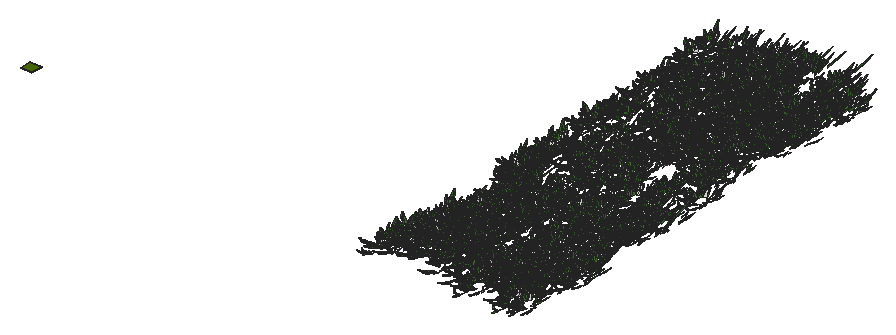
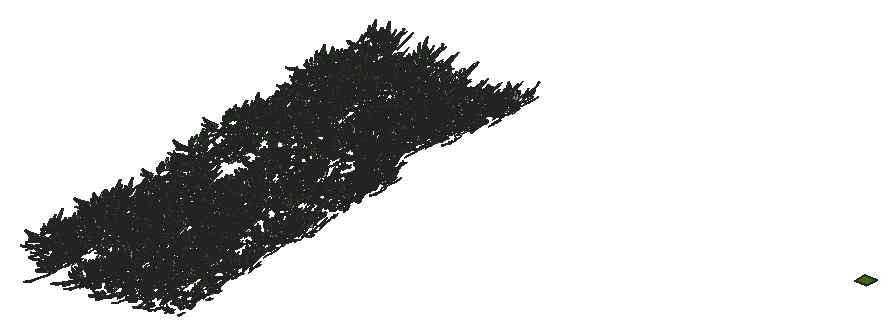
# SketchUp Ruby script. Lengths in inches.
U = 1.inch
M = Sketchup.active_model
def pt(a) = Geom::Point3d.new(a.map { |v| v * U })
def face(e, loops, mat)
  f = e.add_face(loops[0].map { |a| pt(a) })
  loops[1..].each { |l| e.add_face(l.map { |a| pt(a) }).erase! }
  f.material = f.back_material = mat if mat
  f
end
# faces: each face lists its corners as indices into pts; further lists are holes
def faces(e, pts, list, mat = nil) = list.each { |f| face(e, (f[0].is_a?(Array) ? f : [f]).map { |l| l.map { |i| pts[i] } }, mat) }
# xy, xz, yz: faces in a plane at the given z, y or x. An outline is a flat list of corners, or four numbers for a rectangle; further outlines are holes
def ring(l) = l.size == 4 ? [[l[0], l[1]], [l[2], l[1]], [l[2], l[3]], [l[0], l[3]]] : l.each_slice(2).to_a
def flat(e, list, mat, &to3) = list.each { |f| face(e, (f[0].is_a?(Array) ? f : [f]).map { |l| ring(l).map { |u, v| to3.(u, v) } }, mat) }
def xy(e, z, list, mat = nil) = flat(e, list, mat) { |x, y| [x, y, z] }
def xz(e, y, list, mat = nil) = flat(e, list, mat) { |x, z| [x, y, z] }
def yz(e, x, list, mat = nil) = flat(e, list, mat) { |y, z| [x, y, z] }
def lines(e, pts, list) = list.each { |a, b| e.add_line(pt(pts[a]), pt(pts[b])) }
# prism: a flat outline (further loops are holes) pulled along v
def prism(e, loops, v, mat = nil)
  f = face(e, loops, mat); d = Geom::Vector3d.new(v.map { |x| x * U })
  f.pushpull(f.normal.samedirection?(d) ? d.length : -d.length)
end
def box(e, o, s, mat = nil) = prism(e, [[o, [o[0] + s[0], o[1], o[2]], [o[0] + s[0], o[1] + s[1], o[2]], [o[0], o[1] + s[1], o[2]]]], [0, 0, s[2]], mat)
def at(x, y, z, deg = 0) = Geom::Transformation.translation(pt([x, y, z])) * Geom::Transformation.rotation(ORIGIN, Z_AXIS, deg.degrees)
def axes(o, x, y, z) = Geom::Transformation.new([*x, 0, *y, 0, *z, 0, *pt(o).to_a, 1])
def part(name) = M.definitions.add(name)
# library, detail: a bought-in or finely detailed component or shape, given as its bounding box
def library(name, o, s) = part(name).tap { |d| box(d.entities, o, s) }
def detail(e, o, s) = box(e.add_group.entities, o, s)
def put(e, d, t, mat = nil) = e.add_instance(d, t).tap { |i| i.material = mat if mat }
def group(e, t, mat = nil) = e.add_group.tap { |g| g.transformation = t; g.material = mat if mat }.entities
root = M.entities
M.materials.add("Material10").color = [48, 90, 38]
M.materials.add("Material11").color = [68, 110, 48]
M.materials.add("Material12").color = [48, 90, 48]
M.materials.add("Material13").color = [58, 110, 58]
M.materials.add("Material14").color = [58, 90, 38]
M.materials.add("Material15").color = [68, 100, 58]
M.materials.add("Material16").color = [48, 100, 38]
M.materials.add("Material9").color = [68, 110, 58]
M.materials.add("[Groundcover_BarkChips]").color = [80, 57, 35]
M.materials.add("[Groundcover_RiverRock_4inch]").color = [80, 57, 35]
M.materials.add("[Groundcover_Rock_Crushed_2inch]").color = [74, 111, 8]
c1 = part("Untitled")
xy(c1.entities,0.3125,[[-290.45,43.1875,-283.67,49.67]],"[Groundcover_RiverRock_4inch]")
xy(c1.entities,0.6875,[[-290.45,43.1875,-283.67,49.67]],"[Groundcover_Rock_Crushed_2inch]")
xz(c1.entities,43.1875,[[-290.45,0.3125,-283.67,0.6875]],"[Groundcover_BarkChips]")
xz(c1.entities,49.67,[[-290.45,0.3125,-283.67,0.6875]],"[Groundcover_BarkChips]")
yz(c1.entities,-290.45,[[43.1875,0.3125,49.67,0.6875]],"[Groundcover_BarkChips]")
yz(c1.entities,-283.67,[[43.1875,0.3125,49.67,0.6875]],"[Groundcover_BarkChips]")
c2 = part("grass00")
p = [[-0.6875,0.15,0],[-0.56,0.08,5.52],[-0.04,0.03,2.76],[0.48,-0.02,0],[0.35,-0.02,5.52],[-0.1,-0.14,5.52],
  [-0.12,0.65,8.37],[-0.42,0.65,8.37]]
faces(c2.entities,p,[[0,1,2,3],[3,2,4],[1,5,2],[5,4,2],[1,6,5],[4,5,6],[7,6,1]])
c3 = part("Group16\#1")
put(c3.entities,c2,axes([1.44,-0.61,-0.01],[0.05352,0.12609,0],[-0.10704,0.04543,0.07239],[0.06664,-0.02828,0.11628]),"Material12")
put(c3.entities,c2,axes([0.76,-0.15,-0.01],[0.04676,0.24062,0],[-0.23162,0.04501,0.06642],[0.0652,-0.01267,0.23595]),"Material9")
put(c3.entities,c2,axes([0.79,0.01,-0.01],[-0.00606,0.34651,0],[-0.34381,-0.00602,0.0432],[0.04319,0.00076,0.34386]))
put(c3.entities,c2,axes([1,0.23,-0.01],[-0.07192,0.31144,0],[-0.28722,-0.06632,0.1236],[0.12043,0.02781,0.29478]),"Material11")
put(c3.entities,c2,axes([1.66,0.77,-0.01],[-0.13828,0.29651,0],[-0.21551,-0.1005,0.22471],[0.20365,0.09498,0.23779]),"Material16")
put(c3.entities,c2,axes([0.6875,0.52,-0.01],[-0.18126,0.24051,0],[-0.22746,-0.17142,0.09788],[0.07817,0.05891,0.28481]),"Material11")
put(c3.entities,c2,axes([0.68,0.78,-0.01],[-0.215,0.18688,0],[-0.12385,-0.14248,0.21334],[0.13995,0.16101,0.18878]),"Material9")
put(c3.entities,c2,axes([0.56,1,-0.01],[-0.13756,0.07624,0],[-0.06159,-0.11112,0.0927],[0.04494,0.08108,0.12705]),"Material11")
put(c3.entities,c2,axes([0.2,0.64,-0.01],[-0.23729,0.07254,0],[-0.05711,-0.18681,0.153],[0.04473,0.14632,0.19535]),"Material16")
put(c3.entities,c2,axes([0.0625,0.72,-0.01],[-0.28874,0.02525,0],[-0.02179,-0.24916,0.14647],[0.01276,0.14591,0.25012]),"Material9")
put(c3.entities,c2,axes([-0.08,0.62,-0.01],[-0.34089,-0.04187,0],[0.03255,-0.26504,0.216],[-0.02633,0.21439,0.26703]),"Material16")
put(c3.entities,c2,axes([-0.34,0.98,-0.01],[-0.14314,-0.0493,0],[0.04397,-0.12769,0.06843],[-0.02228,0.0647,0.13505]),"Material16")
put(c3.entities,c2,axes([-0.87,1.45,-0.01],[-0.23488,-0.14114,0],[0.13761,-0.22901,0.06087],[-0.03135,0.05217,0.26717]))
put(c3.entities,c2,axes([-0.72,0.77,-0.01],[-0.14208,-0.13251,0],[0.07209,-0.0773,0.16301],[-0.11118,0.11922,0.1057]),"Material16")
put(c3.entities,c2,axes([-0.62,0.43,-0.01],[-0.14845,-0.21203,0],[0.18654,-0.13061,0.12304],[-0.10079,0.07057,0.22772]),"Material9")
put(c3.entities,c2,axes([-0.68,0.29,-0.01],[-0.13639,-0.32136,0],[0.31723,-0.13464,0.05579],[-0.05136,0.0218,0.34462]),"Material10")
put(c3.entities,c2,axes([-0.64,0.125,-0.01],[-0.0458,-0.23569,0],[0.22124,-0.043,0.08276],[-0.08124,0.01579,0.22538]),"Material13")
put(c3.entities,c2,axes([-1.6,-0.03,-0.01],[0.00576,-0.32897,0],[0.27526,0.00482,0.18018],[-0.18015,-0.00315,0.2753]),"Material11")
put(c3.entities,c2,axes([-1.36,-0.31,-0.01],[0.05718,-0.24765,0],[0.18172,0.04196,0.17267],[-0.16825,-0.03885,0.1865]),"Material16")
put(c3.entities,c2,axes([-1.54,-0.72,-0.01],[0.06537,-0.14017,0],[0.13555,0.06321,0.03939],[-0.0357,-0.01665,0.14956]))
put(c3.entities,c2,axes([-1.19,-0.9,-0.01],[0.09597,-0.12735,0],[0.11214,0.08451,0.07557],[-0.06035,-0.04548,0.14042]),"Material15")
put(c3.entities,c2,axes([-0.47,-0.54,-0.01],[0.11588,-0.10072,0],[0.0618,0.0711,0.12124],[-0.07953,-0.0915,0.0942]))
put(c3.entities,c2,axes([-0.47,-0.84,-0.01],[0.11927,-0.0661,0],[0.06603,0.11913,0.00646],[-0.00313,-0.00565,0.13621]),"Material11")
put(c3.entities,c2,axes([-0.38,-1.24,-0.01],[0.28037,-0.08571,0],[0.0618,0.20215,0.20315],[-0.05939,-0.19428,0.21139]),"Material15")
put(c3.entities,c2,axes([-0.06,-0.66,-0.01],[0.22719,-0.01987,0],[0.01247,0.14255,0.17758],[-0.01547,-0.17691,0.1431]),"Material14")
put(c3.entities,c2,axes([0.11,-0.89,-0.01],[0.14882,0.01828,0],[-0.01058,0.08611,0.12229],[0.01491,-0.12138,0.08676]),"Material12")
put(c3.entities,c2,axes([0.25,-0.72,-0.01],[0.20481,0.07053,0],[-0.06206,0.18022,0.10291],[0.03351,-0.0973,0.1906]),"Material12")
put(c3.entities,c2,axes([0.85,-1.42,-0.01],[0.16481,0.09904,0],[-0.09472,0.15762,0.05616],[0.02893,-0.04814,0.18389]),"Material11")
put(c3.entities,c2,axes([1.01,-1.09,-0.01],[0.21858,0.20385,0],[-0.17495,0.1876,0.15339],[0.10462,-0.11218,0.25652]),"Material16")
put(c3.entities,c2,axes([1.01,-0.71,-0.01],[0.08733,0.12473,0],[-0.06445,0.04512,0.13037],[0.1068,-0.07477,0.07867]),"Material12")
c4 = part("Group15\#1")
put(c4.entities,c3,at(0,0,0))
c5 = part("3darcstudiotree_grass00\#1")
put(c5.entities,c4,at(0,0,0))
put(root,c1,at(865.12,488.43,12.75))
put(root,c5,axes([800.23,508.89,12.99],[2.09672,-5.29532,0],[2.32944,4.81953,-0.01132],[0.03564,0.07375,1.83032]))
put(root,c5,axes([800.95,655.86,12.99],[0.31946,-6.70792,0],[3.10987,0.77388,-0.01362],[0.04886,0.01216,1.54899]))
put(root,c5,axes([801.36,701.5,12.99],[-1.12933,-6.15608,0],[2.41129,-2.31138,-0.00949],[0.03992,-0.03827,1.63563]))
put(root,c5,axes([800.76,739.52,12.99],[-1.09212,5.80129,0],[-2.59208,-2.54976,-0.01574],[-0.06215,-0.06113,1.66349]))
put(root,c5,axes([801.09,602.27,12.99],[2.14192,-4.884,0],[1.79828,4.12087,-0.0036],[0.0115,0.02635,1.5794]))
put(root,c5,axes([801.25,727.03,12.99],[-1.91744,4.33181,0],[-2.27081,-5.25216,-0.01852],[-0.0442,-0.10223,1.50457]))
put(root,c5,axes([801.03,526.67,12.99],[2.9199,-1.29353,0],[0.61218,7.22061,-0.01483],[0.00967,0.114,1.51152]))
put(root,c5,axes([802.77,513.77,12.99],[3.12278,0.02412,0],[-0.00853,5.77007,-0.00416],[-0.00005,0.03676,1.3392]))
put(root,c5,axes([804.21,703.32,12.99],[-0.82802,-6.3908,0],[2.45507,-1.66208,-0.01669],[0.08291,-0.05613,1.82011]))
put(root,c5,axes([804.46,691.14,12.99],[-2.76923,-1.21771,0],[0.5023,-5.96879,-0.01319],[0.01203,-0.14291,1.76124]))
put(root,c5,axes([804.6875,601.86,12.99],[1.26765,-5.25445,0],[2.71341,3.42052,-0.00061],[0.00243,0.00307,1.94394]))
put(root,c5,axes([804.25,627.625,12.99],[-1.44997,6.09404,0],[-2.85681,-3.55173,-0.01158],[-0.03373,-0.04193,1.47884]))
put(root,c5,axes([805.29,654.14,12.99],[-0.35039,-7.84154,0],[2.81713,-0.65775,-0.01024],[0.04794,-0.01119,1.82793]))
put(root,c5,axes([804.41,665.98,12.99],[-0.1649,5.55571,0],[-3.24156,-0.50275,-0.00038],[-0.00124,-0.00019,1.44006]))
put(root,c5,axes([804.86,617.52,12.99],[-1.64639,6.87327,0],[-3.05198,-3.81993,-0.00813],[-0.01971,-0.02467,1.31962]))
put(root,c5,axes([805.4,546.16,12.99],[2.54263,-5.12999,0],[2.27143,5.88263,-0.00351],[0.00793,0.02054,1.60808]))
put(root,c5,axes([806.83,619.66,12.99],[-0.74564,-6.43784,0],[2.77952,-1.68216,-0.00114],[0.00493,-0.00299,1.77079]))
put(root,c5,axes([806.68,607.52,12.99],[-2.04166,3.60381,0],[-1.7787,-5.26535,-0.02049],[-0.04461,-0.13206,1.42185]))
put(root,c5,axes([807.05,674.68,12.99],[1.57836,-5.54635,0],[2.22661,3.31092,-0.01966],[0.0743,0.11048,1.64285]))
put(root,c5,axes([807.12,534.26,12.99],[3.12,-0.69524,0],[0.32883,7.71062,-0.00515],[0.00195,0.04561,1.80879]))
put(root,c5,axes([808.6875,521.33,12.99],[-3.07687,-0.64665,0],[0.26983,-6.7085,-0.01686],[0.00528,-0.13122,1.38194]))
put(root,c5,axes([807.71,592.73,12.99],[-0.49105,5.68398,0],[-3.31159,-1.4949,-0.01512],[-0.05957,-0.02689,1.85999]))
put(root,c5,axes([808.86,554.79,12.99],[0.69706,-6.0748,0],[2.812,1.68601,-0.01105],[0.04084,0.02449,1.52421]))
put(root,c5,axes([807.8,515.63,12.99],[0.68888,7.19836,0],[-2.68703,1.34365,-0.00261],[-0.01128,0.00564,1.6704]))
put(root,c5,axes([808.15,597.61,12.99],[-0.05572,7.22617,0],[-3.2808,-0.13219,-0.00958],[-0.03157,-0.00127,1.48335]))
put(root,c5,axes([808.77,545.52,12.99],[0.23357,6.43138,0],[-2.5775,0.48913,-0.00998],[-0.03782,0.00718,1.34846]))
put(root,c5,axes([811.41,619.29,12.99],[-1.01901,-6.34011,0],[2.37512,-1.99468,-0.02344],[0.085,-0.07139,1.34096]))
put(root,c5,axes([811.29,745.75,12.99],[-2.7993,0.80527,0],[-0.3245,-5.89421,-0.01354],[-0.00672,-0.12206,1.41676]))
put(root,c5,axes([811.24,543.27,12.99],[-2.65319,1.41559,0],[-0.56092,-5.49331,-0.0198],[-0.01964,-0.19232,1.47686]))
put(root,c5,axes([811.75,596.32,12.99],[-3.14299,2.69096,0],[-0.86519,-5.2802,-0.01358],[-0.0208,-0.12694,1.47772]))
put(root,c5,axes([812.16,582.22,12.99],[-2.72081,-1.30427,0],[0.6495,-7.07971,-0.00999],[0.00653,-0.07119,1.38276]))
put(root,c5,axes([812.25,533.61,12.99],[2.19634,-5.09007,0],[1.94843,4.39305,-0.00165],[0.00568,0.0128,1.81884]))
put(root,c5,axes([813.18,563.3125,12.99],[-2.5172,-0.31712,0],[0.16715,-6.9327,-0.00601],[0.00142,-0.05907,1.79325]))
put(root,c5,axes([813.24,708.21,12.99],[0.80823,-6.76813,0],[3.05751,1.90783,-0.00598],[0.01798,0.01122,1.35627]))
put(root,c5,axes([812.71,705,12.99],[2.46759,-4.37669,0],[1.49917,4.41653,-0.00126],[0.00308,0.00909,1.3431]))
put(root,c5,axes([812.58,719.11,12.99],[2.65855,-0.90341,0],[0.46643,7.17225,-0.00967],[0.00463,0.07116,1.41667]))
put(root,c5,axes([812.65,665.33,12.99],[1.37674,6.63093,0],[-2.52949,2.7442,-0.01135],[-0.04821,0.05231,1.80626]))
put(root,c5,axes([814.68,523.04,12.99],[2.82554,-3.02642,0],[1.33972,6.53566,-0.00986],[0.01321,0.06445,1.36783]))
put(root,c5,axes([814.94,562.6875,12.99],[-1.03388,7.1157,0],[-2.79608,-2.1228,-0.00679],[-0.02085,-0.01583,1.30662]))
put(root,c5,axes([816.85,637.65,12.99],[-2.85025,-2.62132,0],[1.02288,-5.81158,-0.02256],[0.03478,-0.19762,1.55256]))
put(root,c5,axes([815.54,586.4,12.99],[1.91909,6.16388,0],[-2.12278,3.45343,-0.01154],[-0.03467,0.05641,1.31865]))
put(root,c5,axes([817.53,720.2,12.99],[-2.39108,-4.65865,0],[1.65388,-4.43549,-0.02002],[0.0484,-0.1298,1.30322]))
put(root,c5,axes([816.74,516.16,12.99],[1.31742,5.38877,0],[-2.29242,2.92842,-0.02391],[-0.08644,0.11042,1.49173]))
put(root,c5,axes([816.75,579.49,12.99],[0.48151,7.34676,0],[-3.28997,1.12669,-0.01905],[-0.06482,0.0222,1.57029]))
put(root,c5,axes([819.17,647.41,12.99],[-2.25448,-4.80359,0],[2.15037,-5.2735,-0.00052],[0.00147,-0.0036,1.79691]))
put(root,c5,axes([819.18,731.33,12.99],[0.63706,-5.72894,0],[2.51593,1.46187,-0.00558],[0.02547,0.0148,1.6757]))
put(root,c5,axes([819.12,699.17,12.99],[1.37686,-5.51275,0],[2.6159,3.41387,-0.00497],[0.01417,0.0185,1.35772]))
put(root,c5,axes([819.42,740.91,12.99],[-0.88021,6.7415,0],[-2.4242,-1.65389,-0.00408],[-0.01562,-0.01065,1.38631]))
put(root,c5,axes([820.59,562.74,12.99],[-0.00356,-6.66433,0],[3.43318,-0.00958,-0.02113],[0.06358,-0.00018,1.41674]))
put(root,c5,axes([819.6,532.41,12.99],[2.5667,-1.31506,0],[0.55424,5.65243,-0.01015],[0.00987,0.10068,1.54623]))
put(root,c5,axes([819.58,541,12.99],[-0.93392,5.91904,0],[-2.61844,-2.15876,-0.00809],[-0.0359,-0.0296,1.80065]))
put(root,c5,axes([820.05,569.5625,12.99],[2.17436,-3.88519,0],[1.98974,5.81862,-0.00613],[0.01489,0.04354,1.74641]))
put(root,c5,axes([819.51,623.69,12.99],[0.08746,5.89923,0],[-2.58973,0.20061,-0.00216],[-0.01068,0.00083,1.758]))
put(root,c5,axes([820.24,552.33,12.99],[-2.07777,4.36694,0],[-2.15772,-5.36441,-0.0061],[-0.0173,-0.04302,1.83281]))
put(root,c5,axes([820.24,689.71,12.99],[3.22616,0.60511,0],[-0.20394,5.68137,-0.01884],[-0.00618,0.17211,1.37151]))
put(root,c5,axes([820.34,517.86,12.99],[2.8928,2.85621,0],[-1.02524,5.42573,-0.02193],[-0.03605,0.19077,1.47013]))
put(root,c5,axes([822.89,676.57,12.99],[-1.20636,-5.55105,0],[2.7125,-3.08017,-0.01655],[0.06381,-0.07245,1.78815]))
put(root,c5,axes([823.56,578.02,12.99],[-0.58897,-7.02756,0],[2.48716,-1.08918,-0.01579],[0.06482,-0.02838,1.45182]))
put(root,c5,axes([823.54,587.31,12.99],[-2.4379,5.44598,0],[-1.86779,-4.3689,-0.01484],[-0.05244,-0.12267,1.85373]))
put(root,c5,axes([823.64,615.85,12.99],[1.84036,-4.91055,0],[2.16719,4.24401,-0.00664],[0.01907,0.03735,1.48048]))
put(root,c5,axes([822.96,686.0625,12.99],[0.48089,7.38769,0],[-2.53639,0.86269,-0.01524],[-0.08141,0.02769,1.90022]))
put(root,c5,axes([823.42,718.37,12.99],[1.97484,3.35801,0],[-1.48884,4.57511,-0.0148],[-0.04983,0.15313,1.93047]))
put(root,c5,axes([824.07,544.96,12.99],[-0.41732,6.08263,0],[-2.58911,-0.92819,-0.01794],[-0.07868,-0.02821,1.59592]))
put(root,c5,axes([824.35,742.09,12.99],[0.91111,5.86152,0],[-2.48899,2.02156,-0.0026],[-0.00992,0.00806,1.46428]))
put(root,c5,axes([824.62,552.33,12.99],[0.58399,6.2494,0],[-3.15304,1.53959,-0.00171],[-0.0066,0.00322,1.74655]))
put(root,c5,axes([825.05,530.83,12.99],[2.46454,1.40932,0],[-0.81989,7.49183,-0.00744],[-0.00546,0.04988,1.4009]))
put(root,c5,axes([827.08,719.46,12.99],[-3.08693,0.39887,0],[-0.16162,-6.53595,-0.00256],[-0.00063,-0.02533,1.70382]))
put(root,c5,axes([827.63,689.68,12.99],[-0.60519,-6.22237,0],[2.81212,-1.42913,-0.01455],[0.04905,-0.02493,1.36448]))
put(root,c5,axes([828.4,523.2,12.99],[-3.11946,1.49974,0],[-0.64099,-6.96666,-0.01674],[-0.01464,-0.15909,1.81501]))
put(root,c5,axes([827.49,664.49,12.99],[-0.17209,6.02578,0],[-2.7945,-0.41701,-0.01044],[-0.04083,-0.00609,1.50484]))
put(root,c5,axes([827.41,543.76,12.99],[2.42238,3.11452,0],[-1.46707,5.96221,-0.00275],[-0.00452,0.01835,1.37565]))
put(root,c5,axes([827.91,672.86,12.99],[-1.31888,5.91859,0],[-3.06509,-3.5689,-0.01882],[-0.05302,-0.06173,1.49212]))
put(root,c5,axes([829.24,700.36,12.99],[0.20359,-6.82047,0],[3.44804,0.53779,-0.02398],[0.06601,0.0103,1.30813]))
put(root,c5,axes([828.93,737.32,12.99],[-3.02512,2.60645,0],[-0.97506,-5.91328,-0.00238],[-0.00292,-0.01771,1.31717]))
put(root,c5,axes([829.52,619.9375,12.99],[-0.82036,-5.64423,0],[2.43367,-1.84828,-0.00285],[0.01487,-0.01129,1.93438]))
put(root,c5,axes([829.67,639.47,12.99],[-2.84768,-0.86391,0],[0.43438,-7.48167,-0.01228],[0.00584,-0.10063,1.63767]))
put(root,c5,axes([829.7,644.53,12.99],[-1.23297,4.80723,0],[-2.64304,-3.54216,-0.01566],[-0.05203,-0.06974,1.61828]))
put(root,c5,axes([829.78,532.89,12.99],[2.7385,-3.70952,0],[1.24815,4.81467,-0.02001],[0.05217,0.20125,1.71774]))
put(root,c5,axes([832.11,702.72,12.99],[0.17403,-6.85679,0],[2.88676,0.38285,-0.02273],[0.08601,0.01141,1.50351]))
put(root,c5,axes([832.98,639.82,12.99],[-3.08233,-3.78375,0],[1.37176,-5.83901,-0.02099],[0.03722,-0.15844,1.49075]))
put(root,c5,axes([831.61,746.71,12.99],[2.17693,2.59154,0],[-1.51198,6.63646,-0.0178],[-0.02396,0.10516,1.30843]))
put(root,c5,axes([832.36,601.36,12.99],[2.51758,0.46037,0],[-0.25773,7.36456,-0.00093],[-0.00023,0.00644,1.35201]))
put(root,c5,axes([832.15,543.71,12.99],[2.9588,3.12499,0],[-1.13849,5.63247,-0.00765],[-0.01175,0.05815,1.36419]))
put(root,c5,axes([833.69,524.66,12.99],[-3.08358,-2.23785,0],[0.91471,-6.58588,-0.0262],[0.02604,-0.18751,1.36239]))
put(root,c5,axes([832.41,614.46,12.99],[-0.21246,5.63329,0],[-3.26922,-0.64428,-0.00545],[-0.02341,-0.00461,1.93955]))
put(root,c5,axes([832.54,680.98,12.99],[2.46524,5.03543,0],[-1.98482,5.0775,-0.00121],[-0.00295,0.00754,1.48985]))
put(root,c5,axes([834,587.76,12.99],[-2.85669,-0.34235,0],[0.13176,-5.74497,-0.00586],[0.00152,-0.06641,1.71352]))
put(root,c5,axes([832.95,570.96,12.99],[0.56671,7.35658,0],[-2.47604,0.99666,-0.02162],[-0.08161,0.03285,1.32159]))
put(root,c5,axes([833.54,511.39,12.99],[0.55209,6.09796,0],[-3.20664,1.51699,-0.00233],[-0.00899,0.00425,1.77271]))
put(root,c5,axes([833.875,536.21,12.99],[2.56499,0.38535,0],[-0.20155,7.01003,-0.01423],[-0.00406,0.14106,1.83161]))
put(root,c5,axes([836.48,532.46,12.99],[-1.74375,-6.42168,0],[2.49526,-3.54043,-0.02087],[0.06974,-0.09896,1.58468]))
put(root,c5,axes([836.3,722.47,12.99],[-2.6649,-0.66406,0],[0.34148,-7.16044,-0.01401],[0.00608,-0.12743,1.72979]))
put(root,c5,axes([835.77,671.44,12.99],[2.82099,-0.59633,0],[0.27587,6.81911,-0.00914],[0.0039,0.09647,1.90465]))
put(root,c5,axes([837.8,545.34,12.99],[0.50162,-7.86458,0],[3.38255,1.12732,-0.00277],[0.00875,0.00292,1.49508]))
put(root,c5,axes([836.8,561.62,12.99],[1.62986,5.08793,0],[-2.16042,3.61622,-0.01948],[-0.07376,0.12346,1.72408]))
put(root,c5,axes([838.02,577.31,12.99],[1.47798,-4.49848,0],[2.27881,3.91217,-0.00267],[0.01021,0.01753,1.87177]))
put(root,c5,axes([837.21,571.7,12.99],[2.47383,4.76043,0],[-2.09245,5.68175,-0.01247],[-0.03357,0.09114,1.86292]))
put(root,c5,axes([838,666.84,12.99],[0.04916,6.40106,0],[-3.41589,0.13709,-0.00579],[-0.02267,0.00091,1.83497]))
put(root,c5,axes([839.59,563.6,12.99],[-0.32471,-6.7139,0],[2.51128,-0.63463,-0.00454],[0.02211,-0.00559,1.6986]))
put(root,c5,axes([840.23,714.65,12.99],[-0.76785,-6.80934,0],[2.94546,-1.73553,-0.01269],[0.04988,-0.02939,1.69312]))
put(root,c5,axes([840.27,600.72,12.99],[-0.92517,-5.34084,0],[2.28422,-2.06754,-0.01359],[0.06271,-0.05677,1.67314]))
put(root,c5,axes([840.0625,747.66,12.99],[-3.17981,2.55688,0],[-0.81607,-5.30303,-0.00518],[-0.0095,-0.0617,1.86492]))
put(root,c5,axes([839.83,628.36,12.99],[-2.20203,5.9036,0],[-2.05692,-4.00894,-0.01811],[-0.04833,-0.0942,1.30017]))
put(root,c5,axes([841.05,653.93,12.99],[-3.15553,-0.06216,0],[0.02788,-7.39399,-0.00939],[0.00035,-0.09201,1.9024]))
put(root,c5,axes([840.79,704.21,12.99],[1.59679,-6.72974,0],[2.53447,3.14225,-0.01711],[0.05457,0.06766,1.43496]))
put(root,c5,axes([840.03,577.9,12.99],[2.39367,1.82521,0],[-0.9422,6.45657,-0.00681],[-0.01006,0.06893,1.90695]))
put(root,c5,axes([841.38,646.75,12.99],[0.0902,-7.37071,0],[3.21088,0.20531,-0.00421],[0.01734,0.00111,1.81536]))
put(root,c5,axes([842.12,691.5,12.99],[2.51903,-4.87817,0],[2.06229,5.56456,-0.02128],[0.05043,0.13608,1.60475]))
put(root,c5,axes([841.63,737.11,12.99],[2.03899,3.41743,0],[-1.68284,5.24641,-0.01003],[-0.02079,0.06483,1.36834]))
put(root,c5,axes([842.18,522.86,12.99],[-0.03399,5.62999,0],[-2.72357,-0.08592,-0.02407],[-0.09619,-0.00303,1.49365]))
put(root,c5,axes([844.06,553.68,12.99],[0.0609,-5.70398,0],[2.69835,0.15054,-0.00377],[0.01696,0.00095,1.66719]))
put(root,c5,axes([843.59,664.44,12.99],[3.03294,-1.31512,0],[0.61982,7.46911,-0.00778],[0.00451,0.05441,1.42033]))
put(root,c5,axes([844.66,727.38,12.99],[2.04782,-4.78865,0],[2.06577,4.616,-0.00015],[0.00053,0.00117,1.98495]))
put(root,c5,axes([845.91,722.47,12.99],[-2.33683,-5.95191,0],[2.37176,-4.86569,-0.02493],[0.06079,-0.12471,1.43253]))
put(root,c5,axes([845.72,739.84,12.99],[-3.03971,-1.67502,0],[0.63632,-6.03383,-0.01967],[0.01991,-0.18876,1.60841]))
put(root,c5,axes([845.25,609.43,12.99],[-1.86294,5.81365,0],[-2.00835,-3.36276,-0.02032],[-0.07953,-0.13316,1.65635]))
put(root,c5,axes([844.8,512.3,12.99],[-0.14496,7.16512,0],[-2.91443,-0.30809,-0.00948],[-0.03229,-0.00341,1.36423]))
put(root,c5,axes([846.21,712.09,12.99],[-1.09281,-7.36434,0],[2.53966,-1.96921,-0.01224],[0.06237,-0.04836,1.97883]))
put(root,c5,axes([844.89,672.28,12.99],[1.3619,4.89456,0],[-2.70268,3.92945,-0.00074],[-0.00274,0.00399,1.93092]))
put(root,c5,axes([847.62,747.45,12.99],[-2.94975,-1.75122,0],[0.78993,-6.95242,-0.00758],[0.00759,-0.06684,1.7185]))
put(root,c5,axes([848.17,719.32,12.99],[-0.70162,-7.65767,0],[3.17066,-1.51796,-0.02019],[0.07552,-0.03615,1.69814]))
put(root,c5,axes([848.41,587.01,12.99],[-2.67499,4.25463,0],[-1.60611,-5.27641,-0.01001],[-0.01971,-0.06476,1.32974]))
put(root,c5,axes([849.16,636.28,12.99],[-0.25566,-6.23409,0],[3.02979,-0.64923,-0.00863],[0.02985,-0.0064,1.44957]))
put(root,c5,axes([848.55,625.49,12.99],[3.23481,-2.60197,0],[0.97102,6.30781,-0.0057],[0.00806,0.05233,1.70987]))
put(root,c5,axes([849.34,685.28,12.99],[1.6311,-5.8777,0],[2.1166,3.06914,-0.01781],[0.06568,0.09524,1.50117]))
put(root,c5,axes([849.15,522.36,12.99],[3.16547,-2.84466,0],[0.97801,5.68665,-0.00849],[0.01524,0.08861,1.79934]))
put(root,c5,axes([850.1,663.44,12.99],[0.38939,-6.63436,0],[2.49503,0.76518,-0.00096],[0.00473,0.00145,1.71349]))
put(root,c5,axes([850.08,654.97,12.99],[-2.79892,0.15833,0],[-0.08278,-7.64602,-0.01248],[-0.00092,-0.08529,1.37214]))
put(root,c5,axes([850.12,617.86,12.99],[-2.8002,4.51668,0],[-1.53978,-4.98809,0],[-0.00001,-0.00003,1.91868]))
put(root,c5,axes([850.46,691.23,12.99],[-2.99381,4.11222,0],[-1.30413,-4.96107,-0.02116],[-0.04686,-0.17825,1.49339]))
put(root,c5,axes([851.7,571.23,12.99],[0.10269,-7.75149,0],[3.02443,0.20936,-0.01983],[0.07207,0.00499,1.50947]))
put(root,c5,axes([851.89,712.25,12.99],[-0.51823,-7.16519,0],[3.0573,-1.15541,-0.0168],[0.06047,-0.02285,1.55067]))
put(root,c5,axes([852.16,531.49,12.99],[-2.85782,2.45284,0],[-0.99544,-6.06017,-0.01194],[-0.01852,-0.11272,1.71307]))
put(root,c5,axes([852.89,517.11,12.99],[-2.39587,-3.05528,0],[1.20243,-4.92694,-0.00653],[0.01361,-0.05576,1.4475]))
put(root,c5,axes([853.14,704.17,12.99],[-2.2722,-5.87956,0],[1.90246,-3.84168,-0.00245],[0.00996,-0.02011,1.8862]))
put(root,c5,axes([851.93,615.7,12.99],[-0.34584,5.49826,0],[-2.81888,-0.92647,-0.00494],[-0.01768,-0.00581,1.4129]))
put(root,c5,axes([853.26,542.75,12.99],[0.38914,-7.1838,0],[3.17613,0.89898,-0.00236],[0.00854,0.00242,1.5989]))
put(root,c5,axes([853.11,655.41,12.99],[-2.87812,2.63419,0],[-1.11234,-6.35044,-0.00598],[-0.00921,-0.0526,1.70205]))
put(root,c5,axes([852.35,745.85,12.99],[1.98419,4.20427,0],[-2.27749,5.61635,-0.0132],[-0.031,0.07645,1.58767]))
put(root,c5,axes([853.88,578.57,12.99],[1.22272,5.6698,0],[-2.97246,3.34949,-0.01549],[-0.04343,0.04894,1.42146]))
put(root,c5,axes([855.9,521.39,12.99],[-1.47837,-5.18804,0],[2.69774,-4.01684,-0.00487],[0.01615,-0.02404,1.74651]))
put(root,c5,axes([856.09,533.28,12.99],[0.56789,-5.76047,0],[3.01388,1.55251,-0.02216],[0.07786,0.04011,1.52603]))
put(root,c5,axes([856.55,689.71,12.99],[-3.16631,0.43145,0],[-0.18801,-7.20948,-0.00226],[-0.00058,-0.02234,1.87745]))
put(root,c5,axes([856.36,505.64,12.99],[-2.56666,5.23638,0],[-2.22777,-5.70575,-0.01139],[-0.0292,-0.07479,1.76647]))
put(root,c5,axes([856.5,721.14,12.99],[3.39381,-1.9293,0],[0.62809,5.77314,-0.00031],[0.00036,0.00334,1.72722]))
put(root,c5,axes([856.91,577.44,12.99],[2.55952,-3.74649,0],[1.66876,5.95706,-0.00312],[0.00599,0.0214,1.51309]))
put(root,c5,axes([856.63,590.53,12.99],[3.29329,-1.83684,0],[0.65264,6.1142,-0.01844],[0.02107,0.19742,1.82062]))
put(root,c5,axes([857.33,682.5,12.99],[1.56071,-5.0557,0],[2.31225,3.72975,-0.01427],[0.03935,0.06348,1.30992]))
put(root,c5,axes([857.4,550.3,12.99],[2.00254,-5.52715,0],[2.41596,4.57378,-0.01649],[0.05307,0.10047,1.79785]))
put(root,c5,axes([857.2,702.32,12.99],[0.23945,5.53651,0],[-2.86092,0.64653,-0.01511],[-0.07448,0.01683,1.95375]))
put(root,c5,axes([859.71,654.4,12.99],[0.23138,-5.61808,0],[2.65727,0.57184,-0.01523],[0.08244,0.01774,1.99019]))
put(root,c5,axes([860.37,703.33,12.99],[-0.09172,-6.20041,0],[2.46361,-0.19043,-0.02047],[0.10078,-0.00779,1.66543]))
put(root,c5,axes([860.11,691.89,12.99],[-2.03697,4.99576,0],[-2.30577,-4.9125,-0.00031],[-0.00086,-0.00183,1.61707]))
put(root,c5,axes([861.72,579.64,12.99],[1.06558,-6.88855,0],[2.39469,1.93558,-0.02361],[0.08433,0.06816,1.32009]))
put(root,c5,axes([861.16,662.97,12.99],[0.30363,7.59709,0],[-2.66419,0.55638,-0.02215],[-0.08559,0.01787,1.42375]))
put(root,c5,axes([862.03,676.59,12.99],[0.71307,-7.79401,0],[2.45555,1.17389,-0.01603],[0.06768,0.03236,1.48463]))
put(root,c5,axes([861.3,555.47,12.99],[-0.63634,7.86688,0],[-3.4079,-1.44039,-0.00297],[-0.01162,-0.00491,1.8915]))
put(root,c5,axes([861.24,523.93,12.99],[2.15713,4.66484,0],[-2.08686,5.04241,-0.00432],[-0.01022,0.02469,1.43292]))
put(root,c5,axes([862.28,608.88,12.99],[-1.95191,6.62491,0],[-2.62788,-4.04568,-0.0002],[-0.00074,-0.00113,1.96126]))
put(root,c5,axes([862.51,536.65,12.99],[2.70134,3.39486,0],[-1.42419,5.92148,-0.0244],[-0.0381,0.15839,1.31386]))
put(root,c5,axes([864.28,693.51,12.99],[2.52793,0.94913,0],[-0.43111,5.99966,-0.00501],[-0.00314,0.04369,1.40942]))
put(root,c5,axes([865.9,549.9,12.99],[0.43607,-6.41249,0],[3.02391,1.0745,-0.01704],[0.07241,0.02573,1.80481]))
put(root,c5,axes([865.04,582.84,12.99],[2.81172,0.05119,0],[-0.02115,6.06948,-0.01492],[-0.0006,0.17245,1.84219]))
put(root,c5,axes([865.0625,515.82,12.99],[2.22144,2.73384,0],[-1.19797,5.08643,-0.02125],[-0.0384,0.16303,1.32121]))
put(root,c5,axes([866.34,674.84,12.99],[-1.45728,4.66166,0],[-2.46444,-4.02556,-0.01309],[-0.04021,-0.06568,1.56859]))
put(root,c5,axes([865.83,714.52,12.99],[2.34118,5.26476,0],[-1.75709,4.08276,-0.00671],[-0.02098,0.04876,1.53359]))
put(root,c5,axes([866.48,747.26,12.99],[0.95509,7.30643,0],[-2.36085,1.61255,-0.01522],[-0.05994,0.04094,1.38916]))
put(root,c5,axes([867.87,577.26,12.99],[-3.19396,-0.79529,0],[0.31702,-6.65278,-0.0047],[0.00188,-0.03952,1.4854]))
put(root,c5,axes([866.81,572.09,12.99],[3.00617,3.2705,0],[-1.13935,5.47219,-0.01473],[-0.02598,0.12479,1.49308]))
put(root,c5,axes([868.91,730.28,12.99],[-2.76162,-3.27636,0],[1.32589,-5.83962,-0.02416],[0.04085,-0.17992,1.4491]))
put(root,c5,axes([868.03,533.78,12.99],[0.37711,7.29432,0],[-2.96261,0.80031,-0.00527],[-0.01922,0.00519,1.50433]))
put(root,c5,axes([868.48,741.88,12.99],[2.64985,-0.40535,0],[0.18246,6.23239,-0.02393],[0.00642,0.21931,1.50627]))
put(root,c5,axes([868.38,653.46,12.99],[2.78127,0.91171,0],[-0.37411,5.96342,-0.02285],[-0.01207,0.19236,1.34478]))
put(root,c5,axes([869.59,545.1,12.99],[0.915,-6.76816,0],[2.35333,1.66242,-0.00928],[0.04925,0.03479,1.87692]))
put(root,c5,axes([869.47,709.05,12.99],[1.18119,5.43905,0],[-2.57298,2.9197,-0.01001],[-0.03347,0.03798,1.4706]))
put(root,c5,axes([869.84,624.87,12.99],[2.31925,4.51845,0],[-1.69643,4.54985,-0.00613],[-0.01857,0.04982,1.67562]))
put(root,c5,axes([870.32,618.29,12.99],[1.14452,6.51327,0],[-3.02643,2.77882,-0.00669],[-0.02692,0.02472,1.94122]))
put(root,c5,axes([872.51,511.33,12.99],[-1.44004,-4.51024,0],[2.32046,-3.87128,-0.00015],[0.0006,-0.00101,1.94435]))
put(root,c5,axes([872.5,690.93,12.99],[-2.72604,-1.03911,0],[0.4136,-5.66971,-0.01602],[0.01078,-0.14781,1.41148]))
put(root,c5,axes([873.2,645.51,12.99],[-3.3588,0.77446,0],[-0.26572,-6.02165,-0.00469],[-0.00254,-0.05755,1.96044]))
put(root,c5,axes([873.76,717.29,12.99],[-2.57368,-2.41153,0],[1.19318,-6.65387,-0.01809],[0.02357,-0.13147,1.4829]))
put(root,c5,axes([872.72,673.41,12.99],[2.98206,1.2712,0],[-0.55669,6.8238,-0.00417],[-0.00344,0.04217,1.87295]))
put(root,c5,axes([873.88,586.21,12.99],[-0.52148,-6.75341,0],[2.51692,-1.01552,-0.01992],[0.0897,-0.03619,1.60321]))
put(root,c5,axes([873.54,548.98,12.99],[-2.28742,3.18204,0],[-1.60957,-6.04584,-0.01391],[-0.02943,-0.11056,1.7292]))
put(root,c5,axes([873.45,664.03,12.99],[-1.45511,6.29083,0],[-3.01079,-3.63892,-0.01892],[-0.05244,-0.06338,1.46501]))
put(root,c5,axes([874.74,701.39,12.99],[-2.14515,-4.45599,0],[2.19928,-5.53221,-0.02206],[0.05374,-0.13517,1.62457]))
put(root,c5,axes([873.62,600.68,12.99],[-1.36229,6.60929,0],[-2.73012,-2.94036,-0.00165],[-0.00537,-0.00578,1.48801]))
put(root,c5,axes([874.8,530.82,12.99],[-3.40398,-0.76612,0],[0.3109,-7.21796,-0.00134],[0.0004,-0.00938,1.33719]))
put(root,c5,axes([873.41,685.89,12.99],[1.22791,6.97862,0],[-2.86621,2.63519,-0.0015],[-0.00507,0.00466,1.54039]))
put(root,c5,axes([874.63,606.84,12.99],[0.47234,5.88972,0],[-3.15961,1.32404,-0.00804],[-0.03189,0.01336,1.77733]))
put(root,c5,axes([876.67,532.17,12.99],[-0.75954,-5.9797,0],[2.5309,-1.67977,-0.00444],[0.022,-0.0146,1.86591]))
put(root,c5,axes([877.25,738.11,12.99],[0.19017,-6.25718,0],[2.94563,0.4678,-0.0172],[0.07106,0.01129,1.67763]))
put(root,c5,axes([878.05,567.62,12.99],[-3.21456,1.31811,0],[-0.59042,-7.52376,-0.00093],[-0.00057,-0.00725,1.58752]))
put(root,c5,axes([877.17,525.68,12.99],[2.81551,0.27489,0],[-0.13427,7.18593,-0.01987],[-0.00289,0.15461,1.47043]))
put(root,c5,axes([877.33,588.3,12.99],[2.85968,-1.46641,0],[0.54158,5.51856,-0.00297],[0.00323,0.0329,1.68702]))
put(root,c5,axes([878.58,720.23,12.99],[-2.10734,-2.86587,0],[1.7863,-6.86337,-0.00321],[0.00507,-0.01948,1.48019]))
put(root,c5,axes([878.26,504.09,12.99],[-2.62344,4.98586,0],[-1.8849,-5.18233,-0.00935],[-0.02392,-0.06576,1.61847]))
put(root,c5,axes([877.96,597.1,12.99],[3.1462,-0.07966,0],[0.02927,6.03995,-0.01976],[0.00083,0.17048,1.36845]))
put(root,c5,axes([878.56,704.45,12.99],[1.05604,6.19028,0],[-3.23059,2.87977,-0.01645],[-0.05676,0.05059,1.76201]))
put(root,c5,axes([878.76,639.42,12.99],[0.96183,5.76672,0],[-2.58605,2.25379,-0.01397],[-0.05233,0.04561,1.52193]))
put(root,c5,axes([880.77,583.04,12.99],[-2.64674,-1.70639,0],[0.70831,-5.74063,-0.015],[0.01487,-0.12049,1.30652]))
put(root,c5,axes([880.67,542.8,12.99],[-2.30536,5.80779,0],[-2.15448,-4.46864,-0.0082],[-0.02633,-0.05462,1.73071]))
put(root,c5,axes([881.64,573.53,12.99],[-2.39229,-2.17764,0],[1.27368,-7.31126,-0.01803],[0.02564,-0.14718,1.81493]))
put(root,c5,axes([881.83,695.49,12.99],[-1.17331,-5.13925,0],[2.65356,-3.16554,-0.00435],[0.0141,-0.01683,1.50222]))
put(root,c5,axes([880.81,729.2,12.99],[0.49922,7.32708,0],[-2.4659,0.87789,-0.00889],[-0.03586,0.01277,1.39664]))
put(root,c5,axes([882.58,653.82,12.99],[-2.19543,-2.61499,0],[1.34506,-5.90062,-0.0201],[0.03024,-0.13267,1.30027]))
put(root,c5,axes([881.41,682.1875,12.99],[1.02972,6.65103,0],[-2.5122,2.03232,-0.0171],[-0.08147,0.0659,1.84743]))
put(root,c5,axes([882.57,550.24,12.99],[-0.55499,6.62785,0],[-3.27532,-1.43308,-0.01652],[-0.05339,-0.02336,1.50529]))
put(root,c5,axes([884.65,505.33,12.99],[-2.55773,4.55898,0],[-1.52979,-4.48462,-0.02241],[-0.05964,-0.17484,1.47722]))
put(root,c5,axes([884.51,698.8,12.99],[1.10721,5.5652,0],[-2.45445,2.55157,-0.00419],[-0.01788,0.01859,1.73548]))
put(root,c5,axes([884.78,527.35,12.99],[2.3819,3.52723,0],[-1.6057,5.66576,-0.01048],[-0.02188,0.0772,1.55517]))
put(root,c5,axes([886.36,599.75,12.99],[-3.15564,-3.50536,0],[1.39647,-6.56886,-0.01545],[0.02806,-0.13199,1.8215]))
put(root,c5,axes([884.78,718.53,12.99],[1.96363,6.2271,0],[-2.28909,3.77174,-0.01552],[-0.04684,0.07718,1.43977]))
put(root,c5,axes([885.45,690.96,12.99],[3.16947,-0.51985,0],[0.24334,7.75228,-0.01186],[0.00277,0.08824,1.52253]))
put(root,c5,axes([885.7,549.5,12.99],[-0.98704,7.61034,0],[-2.34307,-1.58789,-0.00114],[-0.00612,-0.00415,1.86907]))
put(root,c5,axes([885.35,586.61,12.99],[0.99229,6.98964,0],[-2.97661,2.20805,-0.01715],[-0.05365,0.0398,1.41194]))
put(root,c5,axes([886.16,626.85,12.99],[-1.40005,5.15389,0],[-2.66644,-3.78483,-0.02009],[-0.0668,-0.09482,1.68525]))
put(root,c5,axes([887.04,730.58,12.99],[-2.21711,6.10539,0],[-2.27694,-4.32047,-0.00469],[-0.01418,-0.02691,1.59556]))
put(root,c5,axes([888.86,536.79,12.99],[-2.15479,4.12792,0],[-2.21416,-6.03929,-0.01682],[-0.04114,-0.11222,1.80026]))
